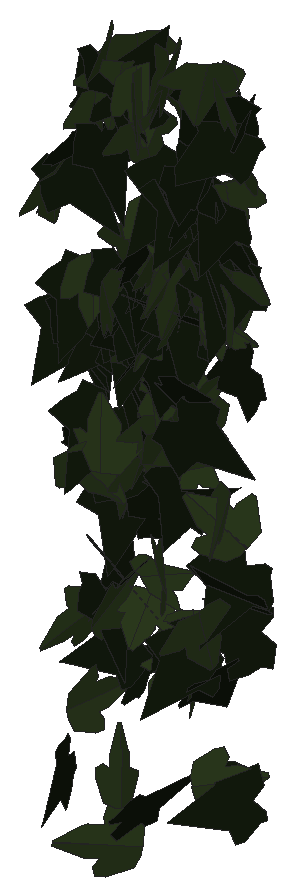
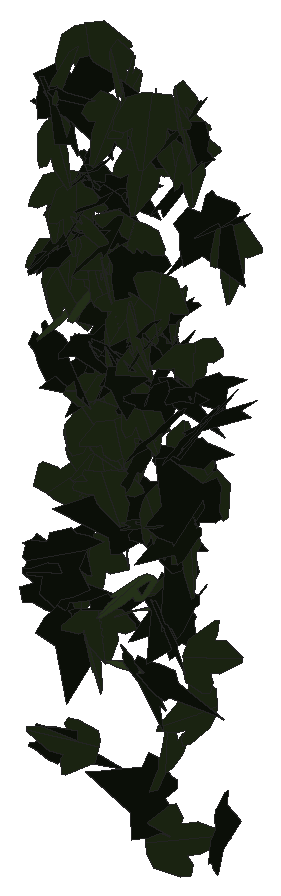
# SketchUp Ruby script. Lengths in inches.
U = 1.inch
M = Sketchup.active_model
def pt(a) = Geom::Point3d.new(a.map { |v| v * U })
def face(e, loops, mat)
  f = e.add_face(loops[0].map { |a| pt(a) })
  loops[1..].each { |l| e.add_face(l.map { |a| pt(a) }).erase! }
  f.material = f.back_material = mat if mat
  f
end
# faces: each face lists its corners as indices into pts; further lists are holes
def faces(e, pts, list, mat = nil) = list.each { |f| face(e, (f[0].is_a?(Array) ? f : [f]).map { |l| l.map { |i| pts[i] } }, mat) }
# xy, xz, yz: faces in a plane at the given z, y or x. An outline is a flat list of corners, or four numbers for a rectangle; further outlines are holes
def ring(l) = l.size == 4 ? [[l[0], l[1]], [l[2], l[1]], [l[2], l[3]], [l[0], l[3]]] : l.each_slice(2).to_a
def flat(e, list, mat, &to3) = list.each { |f| face(e, (f[0].is_a?(Array) ? f : [f]).map { |l| ring(l).map { |u, v| to3.(u, v) } }, mat) }
def xy(e, z, list, mat = nil) = flat(e, list, mat) { |x, y| [x, y, z] }
def xz(e, y, list, mat = nil) = flat(e, list, mat) { |x, z| [x, y, z] }
def yz(e, x, list, mat = nil) = flat(e, list, mat) { |y, z| [x, y, z] }
def lines(e, pts, list) = list.each { |a, b| e.add_line(pt(pts[a]), pt(pts[b])) }
# prism: a flat outline (further loops are holes) pulled along v
def prism(e, loops, v, mat = nil)
  f = face(e, loops, mat); d = Geom::Vector3d.new(v.map { |x| x * U })
  f.pushpull(f.normal.samedirection?(d) ? d.length : -d.length)
end
def box(e, o, s, mat = nil) = prism(e, [[o, [o[0] + s[0], o[1], o[2]], [o[0] + s[0], o[1] + s[1], o[2]], [o[0], o[1] + s[1], o[2]]]], [0, 0, s[2]], mat)
def at(x, y, z, deg = 0) = Geom::Transformation.translation(pt([x, y, z])) * Geom::Transformation.rotation(ORIGIN, Z_AXIS, deg.degrees)
def axes(o, x, y, z) = Geom::Transformation.new([*x, 0, *y, 0, *z, 0, *pt(o).to_a, 1])
def part(name) = M.definitions.add(name)
# library, detail: a bought-in or finely detailed component or shape, given as its bounding box
def library(name, o, s) = part(name).tap { |d| box(d.entities, o, s) }
def detail(e, o, s) = box(e.add_group.entities, o, s)
def put(e, d, t, mat = nil) = e.add_instance(d, t).tap { |i| i.material = mat if mat }
def group(e, t, mat = nil) = e.add_group.tap { |g| g.transformation = t; g.material = mat if mat }.entities
root = M.entities
M.materials.add("efeu1").color = [18, 25, 13]
M.materials.add("efeu2").color = [43, 57, 29]
c1 = part("ivyleaf_9")
p = [[1.54,2.16,1.25],[1.36,2.04,1.19],[-0.21,0.99,0.68],[-0.71,1.11,0.82],[-0.85,0.86,0.67],[-0.8,0.17,0.21],
  [-0.9,-0.01,0.1],[-0.67,-0.16,-0.02],[-0.08,-0.08,-0.05],[-0.03,-0.6,-0.4],[0.65,-0.88,-0.66],[0.83,-0.6,-0.49],
  [1.29,-0.42,-0.43],[1.8125,-0.07,-0.26],[1.21,0.44,0.15]]
faces(c1.entities,p,[[0,1,2,3,4,5,6,7,8,9,10,11,12,13,14]],"efeu1")
c2 = part("ivyleaf_10")
p = [[0,0.5,-0.03],[-0.0625,2.02,-0.43],[-0.19,2.01,-0.46],[-0.54,1.05,-0.29],[-0.52,0.625,-0.18],[-0.83,0.76,-0.28],
  [-1.16,0.64,-0.33],[-1.15,0.33,-0.24],[-0.77,-0.39,0.02],[-0.3,-0.51,0.16],[0.04,-0.48,0.23],[-0.02,2.01,-0.4375],
  [-0.06,2.01,-0.43],[0.04,-0.49,0.23],[0.67,-0.49,0.14],[1.38,0.36,-0.2],[1.375,0.51,-0.24],[0.81,0.65,-0.19],
  [0.62,0.59,-0.15],[0.6,1.09,-0.28],[0.5,1.23,-0.31]]
faces(c2.entities,p,[[0,1,2,3,4,5,6,7,8,9,10],[11,12,0,13,14,15,16,17,18,19,20]],"efeu2")
put(root,c1,axes([589.63,128.55,262.27],[-0.55426,-0.86571,0.42191],[-0.00673,-0.4833,-1.00052],[0.96302,-0.50163,0.23583]))
put(root,c1,axes([589.38,128.5625,262.63],[0.50819,-0.94563,-0.21102],[-0.0284,0.22365,-1.0706],[0.96848,0.50277,0.07933]))
put(root,c1,axes([589.53,128.1,244.55],[-0.0296,-0.2082,-1.05353],[0.86849,-0.62454,0.09902],[-0.63165,-0.84896,0.18552]))
put(root,c2,axes([590.15,126.51,269.06],[-0.08379,-1.13176,-0.31469],[0.00199,0.31535,-1.13467],[1.17469,-0.08126,-0.02053]))
put(root,c1,axes([589.97,128.91,263.83],[-0.59051,-0.92501,0.03891],[0.06784,-0.08926,-1.09238],[0.92334,-0.58502,0.10514]))
put(root,c1,axes([590.62,127.55,270.36],[-0.31932,0.78246,-0.78278],[0.25643,-0.74024,-0.84454],[-1.07667,-0.40837,0.03101]))
put(root,c1,axes([589.91,129.06,261.98],[0.24365,-1.06443,-0.00225],[0.00136,0.00262,-1.09196],[1.06443,0.24365,0.00191]))
put(root,c2,axes([590.93,128.14,256.72],[-0.81051,0.36473,0.68855],[-0.64196,0.2505,-0.88836],[-0.4416,-1.03357,0.02767]))
put(root,c2,axes([590.87,127.625,251.26],[0.02269,-0.34689,1.0574],[-0.00059,-1.05763,-0.34695],[1.11285,0.00651,-0.02174]))
put(root,c2,axes([590.61,128.16,264.8125],[0.57113,0.9593,-0.02444],[-0.00075,-0.028,-1.11636],[-0.95961,0.57097,-0.01368]))
put(root,c1,axes([590.375,126.95,269.62],[0.44722,-0.84391,-0.60624],[0.03777,0.67278,-0.90866],[1.03841,0.33898,0.29415]))
put(root,c1,axes([590.57,128.32,257.43],[0.96775,-0.43318,0.00169],[0.04286,0.09165,-1.05544],[0.43105,0.9634,0.10116]))
put(root,c1,axes([591.69,128.48,262.97],[-1.07107,-0.19623,0.0523],[-0.05344,0.00146,-1.08884],[0.19593,-1.07234,-0.01106]))
put(root,c1,axes([590.59,128.02,257.53],[1.03759,0.33957,-0.26038],[0.24819,0.07878,1.09174],[0.34858,-1.06686,-0.00226]))
put(root,c2,axes([591.5625,127.125,272.46],[-0.01137,-1.11273,0.11096],[0.25307,-0.11065,-1.08366],[1.08923,0.01409,0.25293]))
put(root,c2,axes([591.58,126.38,248.22],[0.03668,-0.10133,1.11114],[-0.05371,1.11029,0.10303],[-1.11445,-0.05685,0.0316]))
put(root,c1,axes([591.4,128.9,253.09],[-0.59195,-0.05492,-0.90653],[0.90765,-0.07337,-0.58823],[-0.03155,-1.08019,0.08604]))
put(root,c1,axes([591.86,127.4,259.8125],[-0.84294,-0.7139,-0.09737],[0.07608,0.06083,-1.10462],[0.71648,-0.84636,0.00274]))
put(root,c1,axes([592.6,128.32,250.23],[-0.96252,0.14666,0.53247],[-0.52389,0.09627,-0.97353],[-0.17485,-1.09577,-0.01426]))
put(root,c2,axes([591.87,127.37,274.75],[0.45316,-1.05296,-0.13502],[-0.01531,0.14031,-1.1456],[1.06148,0.45155,0.04112]))
put(root,c2,axes([591.47,126.42,258.17],[-0.82743,-0.31894,-0.70837],[0.67817,0.20825,-0.88593],[0.37893,-1.06914,0.03875]))
put(root,c1,axes([591.35,127.62,253.95],[1.10339,-0.41949,-0.02096],[-0.01715,0.01385,-1.18043],[0.41966,1.10351,0.00685]))
put(root,c1,axes([591.7,129.2,261.28],[0.03887,-1.05919,0.23083],[0.06094,-0.22848,-1.05866],[1.08233,0.0509,0.05132]))
put(root,c2,axes([592.72,127.33,242.54],[0.0947,0.11164,1.21981],[-0.68837,-1.00712,0.14561],[1.01318,-0.69469,-0.01508]))
put(root,c1,axes([592.82,127.15,264.26],[-0.36494,0.91856,0.47704],[-0.35148,0.36579,-0.97322],[-0.97354,-0.47639,0.17255]))
put(root,c1,axes([592.37,126.97,252.625],[0.21982,0.86274,0.67767],[0.00798,0.68986,-0.88085],[-1.09704,0.17788,0.12938]))
put(root,c1,axes([592.06,129.03,262.83],[-0.47842,-0.97823,-0.09877],[0.04888,0.08604,-1.08894],[0.98199,-0.48088,0.00609]))
put(root,c2,axes([592.39,127.52,273.68],[-0.70005,-0.875,0.19659],[-0.01544,-0.2376,-1.11249],[0.89667,-0.68721,0.13433]))
put(root,c1,axes([591.61,127.63,273.89],[0.60177,-0.96735,-0.0528],[0.08931,0.11728,-1.1309],[0.96466,0.59259,0.13764]))
put(root,c1,axes([592.13,128.52,263.07],[-0.16056,-0.42356,1.01444],[-0.22055,-0.99195,-0.44908],[1.07696,-0.26628,0.05927]))
put(root,c1,axes([592.27,128.11,256.44],[-0.78355,-0.6028,-0.38934],[0.29725,0.25205,-0.98845],[0.65315,-0.83786,-0.01723]))
put(root,c2,axes([592.47,128.05,266.82],[-1.11949,-0.11384,0.02211],[-0.02279,0.00557,-1.12523],[0.11371,-1.11969,-0.00785]))
put(root,c1,axes([591.93,127.12,271.2],[0.31405,-1.09555,-0.11039],[-0.02387,0.10799,-1.13966],[1.10084,0.31488,0.00678]))
put(root,c2,axes([592.38,126.48,258.61],[1.06878,0.30106,0.07668],[-0.08465,0.0179,1.10964],[0.29891,-1.07137,0.04008]))
put(root,c2,axes([592.57,128.35,274.64],[-0.83117,-0.78103,-0.11814],[0.06366,0.1047,-1.14008],[0.78735,-0.83297,-0.03253]))
put(root,c2,axes([592.65,128.83,262.2],[-0.16476,-1.04964,0.22877],[-0.07656,-0.21938,-1.06171],[1.07155,-0.17707,-0.04069]))
put(root,c1,axes([591.98,127.24,252.51],[0.3566,-1.08529,0.1425],[0.05644,-0.13144,-1.1423],[1.09315,0.36082,0.01249]))
put(root,c2,axes([592.54,128.23,257.4],[0.16698,-1.06075,0.22936],[0.08679,-0.21826,-1.07261],[1.08178,0.18124,0.05066]))
put(root,c1,axes([591.8,128.4,257.09],[0.30627,-1.0059,-0.21009],[0.64462,0.35879,-0.77815],[0.80028,0.09596,0.7072]))
put(root,c1,axes([592.2,128,265.54],[0.04848,-1.10628,-0.13717],[0.06604,0.13991,-1.10503],[1.1128,0.0399,0.07156]))
put(root,c2,axes([592.77,126.34,265.38],[-0.31304,0.98969,0.36686],[-0.30291,0.28232,-1.0201],[-1.0111,-0.39099,0.19203]))
put(root,c1,axes([592.44,127.17,272.31],[-0.78587,0.1479,1.03636],[1.02018,-0.18248,0.79964],[0.23482,1.28776,-0.00571]))
put(root,c2,axes([592.9,126,252.45],[0.29035,-0.56349,0.97249],[-0.26476,0.94186,0.62479],[-1.09232,-0.37808,0.10706]))
put(root,c1,axes([593.55,127.64,249.67],[-0.35534,0.78424,0.68069],[-0.35356,0.58508,-0.85866],[-0.9764,-0.49727,0.06321]))
put(root,c2,axes([592.96,128.73,265.74],[0.38067,-1.03113,0.1237],[0.05105,-0.11301,-1.09912],[1.03727,0.38398,0.0087]))
put(root,c2,axes([593.19,126.44,245.32],[-0.11746,1.05571,-0.48115],[-0.04748,0.47883,1.06221],[1.15922,0.12658,-0.00524]))
put(root,c1,axes([592.6,128.69,264.46],[0.01732,-0.82058,0.74143],[0.14891,-0.73304,-0.81477],[1.09585,0.11258,0.099]))
put(root,c1,axes([593.41,129.04,263.4375],[-0.70841,0.4181,-0.72129],[0.40084,-0.65913,-0.77575],[-0.73102,-0.76658,0.27362]))
put(root,c1,axes([592.75,128.87,259.3],[-0.05883,-0.52167,0.94009],[0.23306,-0.9253,-0.49888],[1.04957,0.17622,0.16347]))
put(root,c2,axes([593.29,128.53,263.87],[-0.01814,0.91133,-0.57721],[-0.24021,-0.5662,-0.88641],[-1.05165,0.11361,0.21242]))
put(root,c1,axes([593.78,127.65,267.48],[-0.43633,0.98978,-0.4697],[0.16811,-0.43911,-1.08148],[-1.08261,-0.4671,0.02137]))
put(root,c2,axes([593.51,127.4,271.92],[-0.5539,-0.94917,-0.30611],[0.14227,0.27137,-1.09888],[0.98711,-0.57172,-0.01339]))
put(root,c2,axes([593.28,127.48,273.65],[0.42217,1.08872,0.04324],[0.01896,0.03903,-1.1677],[-1.08941,0.42258,-0.00356]))
put(root,c2,axes([593.17,128.71,266],[-0.96213,-0.21167,-0.50134],[0.53987,-0.24304,-0.93344],[0.06851,-1.05734,0.31492]))
put(root,c2,axes([593.54,127.04,273.62],[-0.45582,1.04116,-0.13566],[-0.11124,-0.19495,-1.12242],[-1.04405,-0.43379,0.17882]))
put(root,c2,axes([593.5,127.75,252.43],[-0.93306,-0.38092,0.23235],[0.35022,-0.95894,-0.16573],[0.27647,-0.07084,0.9941]))
put(root,c1,axes([593.24,127.9,264.09],[0.08342,-0.73778,-0.80673],[0.06055,0.81095,-0.73538],[1.09155,0.01139,0.10245]))
put(root,c1,axes([593.29,126.73,244],[0.10398,1.06265,-0.44322],[0.02821,0.44254,1.06764],[1.15103,-0.10684,0.01387]))
put(root,c2,axes([593.58,127.75,253.53],[0.9006,-0.30499,-0.44926],[0.28389,1.00615,-0.11396],[0.46288,-0.02369,0.94398]))
put(root,c2,axes([593.875,128.66,260.59],[0.68758,0.80245,-0.16364],[-0.12345,-0.10968,-1.0565],[-0.80961,0.69822,0.02211]))
put(root,c2,axes([594.14,127.53,260.04],[-0.46261,-0.96244,0.09659],[-0.02221,-0.09647,-1.06762],[0.96702,-0.46263,0.02168]))
put(root,c2,axes([594.34,128.38,264.17],[0.32748,-1.02109,-0.106],[0.03187,0.12132,-1.07022],[1.02608,0.32212,0.06707]))
put(root,c2,axes([593.95,127.61,268.66],[1.04629,0.36666,0.39342],[0.37202,0.128,-1.10868],[-0.38836,1.11046,-0.00211]))
put(root,c2,axes([594.36,128.69,258.16],[1.00844,0.3806,-0.17497],[-0.16141,-0.06786,-1.07785],[-0.38655,1.02125,-0.00641]))
put(root,c2,axes([594.54,128.28,250.07],[-1.01905,-0.05539,0.04062],[0.04683,-1.00214,-0.19159],[0.05025,-0.1893,1.00241]))
put(root,c1,axes([594.73,128.9,263.91],[-1.0263,-0.17049,-0.26648],[0.27325,-0.02192,-1.03838],[0.1594,-1.06011,0.06432]))
put(root,c2,axes([594.48,127.92,262.22],[0.50419,0.90977,-0.2903],[-0.18381,-0.22968,-1.03904],[-0.9371,0.53453,0.04762]))
put(root,c1,axes([593.875,127.35,256.27],[0.3777,0.2079,1.08516],[0.97077,0.48521,-0.43084],[-0.52764,1.04154,-0.0159]))
put(root,c2,axes([594.98,128.94,260.62],[-0.68513,-0.5885,0.62316],[-0.40147,-0.48451,-0.89896],[0.75729,-0.78929,0.0872]))
put(root,c2,axes([594.35,128.41,266.49],[1.07113,-0.30833,0.11835],[0.14224,0.06817,-1.10974],[0.29807,1.07549,0.10428]))
put(root,c2,axes([594.7,128.2,266.83],[0.53535,-0.98347,-0.09124],[-0.05378,0.07461,-1.11967],[0.98622,0.53792,-0.01153]))
put(root,c2,axes([594.19,127.64,274.09],[0.00412,0.02264,1.17313],[0.73506,-0.91445,0.01506],[0.91456,0.73487,-0.0174]))
put(root,c2,axes([594.64,128.54,258.65],[-0.92135,-0.65919,0.17745],[0.15007,0.0952,1.13284],[-0.66596,0.93344,0.00978]))
put(root,c2,axes([594.35,127.62,259.13],[-0.37552,-0.38786,-0.98717],[0.68611,0.70976,-0.53986],[0.80882,-0.78215,-0.00037]))
put(root,c1,axes([594.54,127.36,262.71],[0.56106,-0.6018,-0.76512],[-0.42416,0.64372,-0.81735],[0.87616,0.697,0.09426]))
put(root,c2,axes([594.65,127.18,259.26],[-0.06262,-1.05409,0.53907],[0.02955,0.53827,1.05595],[-1.18357,0.06921,-0.00216]))
put(root,c2,axes([594.76,127.93,273.49],[-1.08131,0.40401,-0.15754],[0.156,-0.03247,-1.15407],[-0.4046,-1.09224,-0.02396]))
put(root,c1,axes([595.3,128.13,264.32],[-1.08117,-0.04576,0.04978],[0.05006,-1.0778,0.09662],[0.04545,0.09874,1.07781]))
put(root,c1,axes([595.1,127.65,270.24],[-0.93563,-0.64753,0.04356],[-0.00688,-0.06652,-1.13672],[0.64896,-0.93428,0.05075]))
put(root,c1,axes([594.49,127.96,269.16],[0.93375,-0.56346,-0.31017],[-0.26522,0.16081,-1.09058],[0.58596,0.97068,0.00063]))
put(root,c1,axes([594.8,128.84,264.29],[-0.39204,-1.05459,-0.21128],[0.06716,0.20043,-1.12508],[1.07345,-0.39769,-0.00677]))
put(root,c2,axes([595.03,127.24,275.27],[0.484,-1.04479,0.02253],[0.01979,-0.01566,-1.1514],[1.04485,0.48427,0.01137]))
put(root,c2,axes([595.625,125.83,254.91],[0.05456,0.10617,-1.23968],[-0.5576,1.11137,0.07064],[1.11227,0.55194,0.09622]))
put(root,c2,axes([594.98,128.27,251.8],[0.87244,0.63682,-0.05341],[-0.03883,-0.03739,-1.08011],[-0.63787,0.87327,-0.0073]))
put(root,c2,axes([595.1,127.48,267.06],[0.06264,-0.53668,1.05015],[0.33715,-0.99959,-0.53095],[1.13012,0.32795,0.10019]))
put(root,c2,axes([595.36,127.37,266.41],[-0.15915,-1.06257,0.40838],[0.04869,-0.41832,-1.06948],[1.1373,-0.13078,0.10293]))
put(root,c2,axes([595.25,127.4,267.53],[-0.82631,0.6893,-0.25631],[0.17372,-0.19166,-1.0755],[-0.71459,-0.84365,0.03492]))
put(root,c1,axes([595.35,127.84,269.93],[-0.91746,-0.30827,-0.60387],[0.59133,0.13323,-0.96643],[0.33168,-1.09024,0.05265]))
put(root,c1,axes([595.36,127.91,269.46],[-0.53143,-0.92833,0.33304],[0.06087,-0.40846,-1.04144],[0.98438,-0.47591,0.24419]))
put(root,c1,axes([595.1,127.55,257.61],[-0.077,-0.86358,0.65064],[0.10861,-0.65516,-0.85673],[1.07578,0.00433,0.13306]))
put(root,c1,axes([595.43,128.31,268.09],[-0.71821,-0.77799,-0.32497],[0.27472,0.18766,-1.05642],[0.79712,-0.76565,0.07128]))
put(root,c2,axes([595.63,127.34,260.91],[0.10383,-0.51344,0.99573],[-0.17518,0.98025,0.52373],[-1.10653,-0.20337,0.01052]))
put(root,c1,axes([595.21,126.59,262.31],[1.07442,0.25417,0.03851],[0.03906,0.00217,-1.10405],[-0.25409,1.07511,-0.00687]))
put(root,c2,axes([595.74,127.98,250.51],[0.51094,-0.92071,-0.02251],[-0.00711,0.0218,-1.05298],[0.92096,0.51097,0.00436]))
put(root,c2,axes([594.86,128.66,268.01],[0.3462,-0.21402,-1.07935],[1.0351,-0.32055,0.39557],[-0.37333,-1.08725,0.09584]))
put(root,c1,axes([596.45,126.68,270.09],[-0.79458,0.80281,0.0977],[-0.08815,0.05017,-1.12921],[-0.80391,-0.79899,0.02725]))
put(root,c1,axes([596.05,127.35,251.49],[-0.79496,-0.67298,0.20649],[-0.12579,-0.17066,-1.04045],[0.69261,-0.80341,0.04804]))
put(root,c2,axes([596.08,128.35,269.65],[-0.4546,-1.01838,-0.09694],[0.06603,0.07665,-1.11487],[1.02085,-0.45846,0.02894]))
put(root,c1,axes([595.93,126.51,271.5],[0.57186,-0.50748,-0.82242],[-0.41243,0.73606,-0.74097],[0.87396,0.67942,0.18847]))
put(root,c2,axes([596.54,128.45,265.85],[-0.1656,-1.00146,0.40409],[-0.09316,-0.39404,-1.01474],[1.07589,-0.18826,-0.02566]))
put(root,c1,axes([596.91,127.53,274.14],[0.363,0.56089,-0.98218],[-0.56781,-0.80175,-0.6677],[-0.9782,0.67353,0.02311]))
put(root,c1,axes([596.68,127.32,250.61],[0.2408,1.04941,0.05142],[0.01516,0.04928,-1.07668],[-1.05056,0.24125,-0.00375]))
put(root,c1,axes([596.17,128.74,267.69],[-0.00443,-1.10156,0.03885],[0.0037,-0.03887,-1.10156],[1.10224,-0.0043,0.00385]))
put(root,c2,axes([596.79,126.84,275.49],[-0.72909,-0.87195,0.16764],[-0.11048,-0.12615,-1.1366],[0.88101,-0.73741,-0.00379]))
put(root,c2,axes([596.63,128.36,269.91],[-0.78196,-0.78736,-0.14111],[0.17428,0.02489,-1.10468],[0.78069,-0.7942,0.10526]))
put(root,c1,axes([597.41,128.53,263.02],[0.02401,-0.02488,-1.08064],[-1.03264,-0.32,-0.01558],[-0.31948,1.03245,-0.03087]))
put(root,c1,axes([596.27,128.09,268.74],[0.8491,-0.6193,-0.36403],[-0.22092,0.31119,-1.04469],[0.68356,0.86986,0.11456]))
put(root,c2,axes([596.8,126.59,253.36],[-0.43345,-1.11619,-0.35215],[0.16119,0.31501,-1.1969],[1.15927,-0.46114,0.03476]))
put(root,c2,axes([596.27,127.76,264.95],[0.70327,-0.79037,-0.34813],[0.61464,0.77343,-0.51428],[0.60671,0.13262,0.92455]))
put(root,c2,axes([596.02,127.99,245.91],[0.23697,-0.01851,-1.04724],[1.00276,0.31416,0.22135],[0.30255,-1.02673,0.08661]))
put(root,c2,axes([597.53,128,271.74],[-0.65203,0.12835,0.91484],[-0.88305,0.24229,-0.66337],[-0.27133,-1.09698,-0.03948]))
put(root,c2,axes([597.32,127.83,256.45],[0.45289,0.7039,0.76279],[-0.57116,-0.52589,0.8244],[0.86666,-0.71441,0.1447]))
put(root,c1,axes([597,128.79,254.62],[-0.79374,-0.77784,0.00642],[-0.00779,-0.00122,-1.11132],[0.77782,-0.79376,-0.00458]))
put(root,c1,axes([596.62,128.16,269.6],[-0.19778,-1.00435,0.46953],[0.01902,-0.47994,-1.01862],[1.10852,-0.17096,0.10125]))
put(root,c1,axes([596.05,126.46,261.2],[0.16271,-0.19362,-1.10253],[0.80255,0.79686,-0.0215],[0.78037,-0.77914,0.252]))
put(root,c1,axes([597.63,128.3,245.62],[-0.8848,-0.09292,0.56212],[-0.55667,-0.08022,-0.88948],[0.12139,-1.04519,0.01829]))
put(root,c1,axes([597.26,128.74,253.13],[-1.01949,-0.15057,0.08036],[0.16933,-0.95337,0.36181],[0.02141,0.37,0.96495]))
put(root,c2,axes([597.08,127.41,266],[0.92577,-0.49146,-0.36989],[-0.26953,0.27668,-1.04221],[0.55291,0.95777,0.11127]))
put(root,c1,axes([597.42,127.49,272.44],[0.00662,0.55795,1.00845],[-0.20171,0.99346,-0.54834],[-1.13472,-0.17334,0.10335]))
put(root,c2,axes([597.13,128.11,266.68],[-1.08717,-0.09326,0.04684],[-0.04623,-0.00905,-1.09115],[0.09356,-1.08814,0.00506]))
put(root,c1,axes([597.8,128.56,252.46],[-0.3911,-0.48152,-0.92773],[-0.61299,-0.69666,0.62],[-0.84663,0.72685,-0.02034]))
put(root,c1,axes([597.59,127.8,272.94],[-1.09947,-0.29734,0.28822],[-0.26302,-0.13016,-1.13763],[0.31985,-1.12914,0.05524]))
put(root,c1,axes([597.02,128.17,266.89],[-0.45989,-1.03339,-0.02298],[-0.00199,0.02603,-1.13103],[1.03364,-0.45973,-0.0124]))
put(root,c2,axes([597.12,127.46,274.78],[-0.44918,1.07798,0.22484],[-0.06224,0.21758,-1.16754],[-1.09942,-0.45273,-0.02577]))
put(root,c2,axes([597.26,127.24,257.97],[0.78925,-0.81529,-0.0645],[-0.02142,0.069,-1.13427],[0.81756,0.78887,0.03255]))
